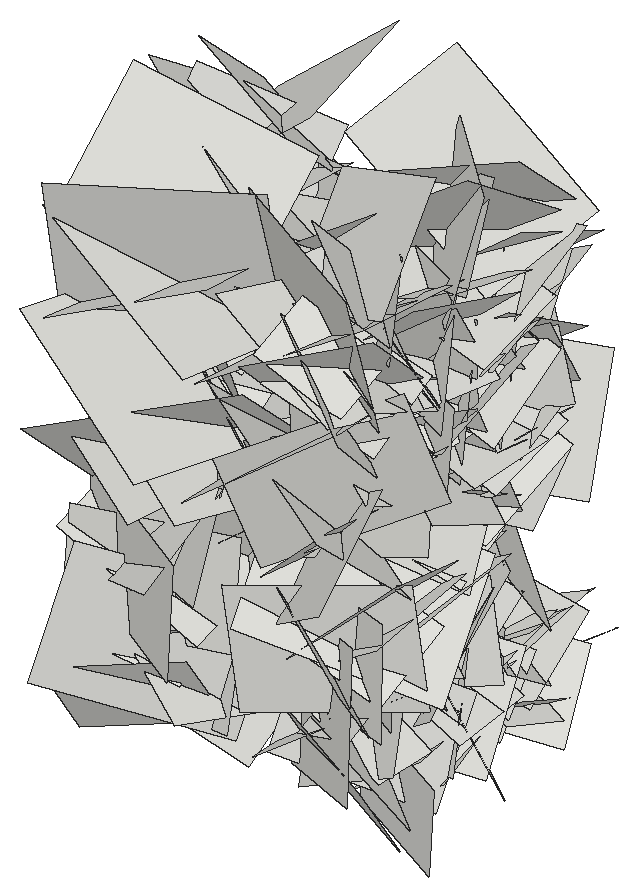
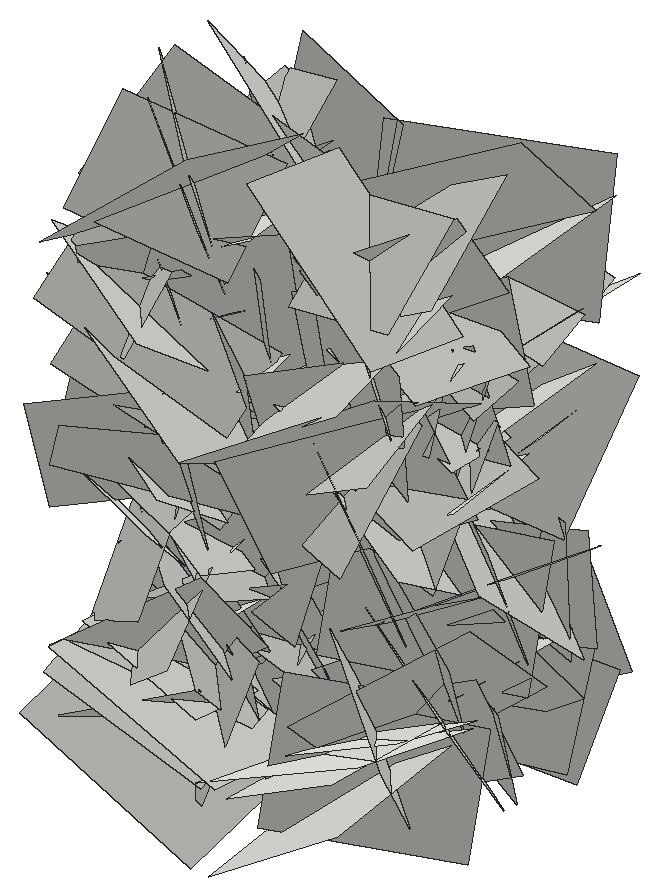
# SketchUp Ruby script. Lengths in inches.
U = 1.inch
M = Sketchup.active_model
def pt(a) = Geom::Point3d.new(a.map { |v| v * U })
def face(e, loops, mat)
  f = e.add_face(loops[0].map { |a| pt(a) })
  loops[1..].each { |l| e.add_face(l.map { |a| pt(a) }).erase! }
  f.material = f.back_material = mat if mat
  f
end
# faces: each face lists its corners as indices into pts; further lists are holes
def faces(e, pts, list, mat = nil) = list.each { |f| face(e, (f[0].is_a?(Array) ? f : [f]).map { |l| l.map { |i| pts[i] } }, mat) }
# xy, xz, yz: faces in a plane at the given z, y or x. An outline is a flat list of corners, or four numbers for a rectangle; further outlines are holes
def ring(l) = l.size == 4 ? [[l[0], l[1]], [l[2], l[1]], [l[2], l[3]], [l[0], l[3]]] : l.each_slice(2).to_a
def flat(e, list, mat, &to3) = list.each { |f| face(e, (f[0].is_a?(Array) ? f : [f]).map { |l| ring(l).map { |u, v| to3.(u, v) } }, mat) }
def xy(e, z, list, mat = nil) = flat(e, list, mat) { |x, y| [x, y, z] }
def xz(e, y, list, mat = nil) = flat(e, list, mat) { |x, z| [x, y, z] }
def yz(e, x, list, mat = nil) = flat(e, list, mat) { |y, z| [x, y, z] }
def lines(e, pts, list) = list.each { |a, b| e.add_line(pt(pts[a]), pt(pts[b])) }
# prism: a flat outline (further loops are holes) pulled along v
def prism(e, loops, v, mat = nil)
  f = face(e, loops, mat); d = Geom::Vector3d.new(v.map { |x| x * U })
  f.pushpull(f.normal.samedirection?(d) ? d.length : -d.length)
end
def box(e, o, s, mat = nil) = prism(e, [[o, [o[0] + s[0], o[1], o[2]], [o[0] + s[0], o[1] + s[1], o[2]], [o[0], o[1] + s[1], o[2]]]], [0, 0, s[2]], mat)
def at(x, y, z, deg = 0) = Geom::Transformation.translation(pt([x, y, z])) * Geom::Transformation.rotation(ORIGIN, Z_AXIS, deg.degrees)
def axes(o, x, y, z) = Geom::Transformation.new([*x, 0, *y, 0, *z, 0, *pt(o).to_a, 1])
def part(name) = M.definitions.add(name)
# library, detail: a bought-in or finely detailed component or shape, given as its bounding box
def library(name, o, s) = part(name).tap { |d| box(d.entities, o, s) }
def detail(e, o, s) = box(e.add_group.entities, o, s)
def put(e, d, t, mat = nil) = e.add_instance(d, t).tap { |i| i.material = mat if mat }
def group(e, t, mat = nil) = e.add_group.tap { |g| g.transformation = t; g.material = mat if mat }.entities
root = M.entities
c1 = part("Component\#6")
p = [[0.01,0,0],[0,3.24,4.54],[4.32,3.24,4.54],[4.33,0,0]]
faces(c1.entities,p,[[0,1,2,3]])
put(root,c1,axes([14.53,197.24,20.32],[0.11105,0.4932,0.81979],[-0.10012,0.82599,-0.48487],[1.00916,0.02768,-0.13831]))
put(root,c1,axes([14.53,196.19,13.89],[-0.03711,0.95345,-0.08325],[0.1071,-0.07916,-0.94908],[1.00884,0.04348,0.09769]))
put(root,c1,axes([18.5,198.53,13.8],[0.10676,-0.41647,0.70694],[0.09382,0.7136,0.40779],[-0.86465,0.02601,0.13154]))
put(root,c1,axes([18.5,201.03,8.02],[0.03451,-0.61291,-0.20918],[-0.0475,-0.21108,0.61149],[-0.68484,-0.01625,-0.05296]))
put(root,c1,axes([18.5,199.53,17.66],[0.07108,0.22718,0.77768],[0.14032,0.76678,-0.23541],[-0.84726,0.14605,0.02626]))
put(root,c1,axes([18.5,196.1,5.28],[0.08762,-0.56519,-0.39893],[-0.0287,-0.4041,0.56691],[-0.73275,-0.05175,-0.06991]))
put(root,c1,axes([14.53,192.44,8.79],[-0.05887,1.04295,0.25043],[0.00297,0.2509,-1.04431],[1.13694,0.05335,0.0157]))
put(root,c1,axes([14.53,193.71,0.46],[0.00413,-0.52236,0.7551],[0.18121,0.74232,0.51263],[0.95624,-0.13842,-0.10041]))
put(root,c1,axes([14.53,195.28,4.79],[0.03702,0.87634,0.85063],[-0.28559,0.83554,-0.84973],[1.26267,0.16329,-0.21713]))
put(root,c1,axes([14.53,203.91,5.3125],[0.18463,-0.58129,-0.78091],[-0.13848,-0.80009,0.56643],[1.02258,-0.00339,0.2177]))
put(root,c1,axes([14.53,198.93,5.125],[0.08676,0.85287,0.14934],[0.16568,0.13299,-0.84515],[0.90272,-0.10637,0.14076]))
put(root,c1,axes([14.53,198.84,9.75],[-0.24721,-0.9594,-0.88495],[-0.06038,-0.89063,0.98057],[1.38221,-0.2105,-0.11544]))
put(root,c1,axes([14.53,202.1,18.26],[-0.1919,-1.13475,-0.09678],[0.16378,-0.12156,1.13628],[1.19604,-0.16542,-0.17113]))
put(root,c1,axes([18.5,194.11,10.49],[0.01019,-0.66626,0.06574],[0.1187,0.06642,0.65679],[-0.69967,0.00157,0.11238]))
put(root,c1,axes([14.53,200.51,5.45],[-0.07717,-0.59417,-0.91785],[0.09928,-0.91989,0.58806],[1.15472,0.03938,-0.1119]))
put(root,c1,axes([14.53,205.24,14.9],[-0.1168,-0.46047,-1.13614],[-0.0362,-1.13913,0.465],[1.29896,-0.07315,-0.0892]))
put(root,c1,axes([14.53,194.25,1.05],[0.1707,-0.55728,0.79671],[-0.04122,0.80323,0.5697],[1.02978,0.12452,-0.10926]))
put(root,c1,axes([14.53,194.35,10.5],[-0.1187,0.07765,-1.12146],[0.14385,-1.11784,-0.09095],[1.18288,0.14373,-0.10148]))
put(root,c1,axes([14.53,197.36,24.8],[-0.09794,1.0389,-0.68546],[-0.01654,-0.68826,-1.04104],[1.31923,0.0685,-0.06394]))
put(root,c1,axes([18.5,199.74,12.37],[0.13977,-0.41949,-0.41774],[-0.0557,-0.43458,0.41982],[-0.62506,-0.05508,-0.13082]))
put(root,c1,axes([18.5,199.42,15.6],[0.03605,-0.49998,-0.38134],[0.14474,-0.36691,0.49324],[-0.65063,-0.10932,0.0886]))
put(root,c1,axes([14.53,200.08,24.34],[0.03463,0.75517,-0.67877],[0.20748,-0.67107,-0.73718],[1.05612,0.10708,0.16708]))
put(root,c1,axes([14.53,199.09,16.39],[0.13116,-1.14374,0.05938],[-0.13174,0.04596,1.1443],[1.20683,0.12933,0.11846]))
put(root,c1,axes([14.53,192.66,5.0625],[0.03803,0.06475,1.02957],[0.25075,1.00223,-0.07127],[1.06436,-0.23842,-0.02]))
put(root,c1,axes([14.53,196.53,2.03],[0.14871,0.38131,0.94323],[0.09041,0.94439,-0.39446],[1.07463,-0.13222,-0.09734]))
put(root,c1,axes([14.53,200.2,14.91],[0.20407,-0.96139,-0.18597],[0.07393,-0.17559,0.97991],[1.03533,0.20204,-0.03331]))
put(root,c1,axes([14.53,198.375,11.05],[-0.00636,-0.47599,-1.14741],[-0.03555,-1.14695,0.47597],[1.31628,-0.03327,0.00731]))
put(root,c1,axes([14.53,202.25,12.93],[-0.19135,-1.27912,0.12446],[0.2118,0.09622,1.27869],[1.34571,-0.19703,-0.18355]))
put(root,c1,axes([14.53,197.86,18.23],[0.19608,0.2602,-1.0463],[-0.01915,-1.06069,-0.26697],[1.14269,-0.06243,0.17507]))
put(root,c1,axes([14.53,197.84,4.84],[0.11369,-0.36766,-0.96616],[0.19069,-0.94989,0.38144],[1.07906,0.2066,0.03439]))
put(root,c1,axes([14.53,200.375,7.61],[0.26418,-0.51362,-0.84712],[0.05211,-0.86603,0.53955],[1.04881,0.1724,0.18657]))
put(root,c1,axes([14.53,203.04,12.11],[0.14841,-0.94408,-0.5752],[0.05434,-0.57362,0.95398],[1.17058,0.14632,0.02864]))
put(root,c1,axes([14.53,199.56,18.73],[0.07364,1.07871,-0.62029],[-0.05176,-0.61841,-1.08091],[1.31797,-0.08456,-0.00779]))
put(root,c1,axes([14.53,204.42,20.53],[0.1154,-1.25003,-0.28156],[-0.14973,-0.29256,1.24425],[1.34995,0.07441,0.16208]))
put(root,c1,axes([14.53,195.93,15.54],[0.04965,0.25406,1.2028],[0.02984,1.20314,-0.25523],[1.30276,-0.03724,-0.03999]))
put(root,c1,axes([14.53,198.85,12.57],[0.15345,0.48368,1.12599],[-0.09378,1.13498,-0.47617],[1.29562,0.02486,-0.16783]))
put(root,c1,axes([14.53,200.7,5.85],[0.20906,1.0682,-0.14016],[0.07965,-0.15578,-1.08152],[1.13921,-0.18514,0.10133]))
put(root,c1,axes([14.53,194.09,6.34],[0.25898,1.07168,-0.21064],[-0.01285,-0.21318,-1.09862],[1.15764,-0.24212,0.03493]))
put(root,c1,axes([14.53,192.7,21.39],[0.08893,0.79245,0.9015],[0.06254,0.89988,-0.79652],[1.27076,-0.09974,-0.02389]))
put(root,c1,axes([14.53,199.38,-0.0625],[0.15183,-0.50198,1.07326],[0.00307,1.08122,0.50532],[1.25594,0.05804,-0.13098]))
put(root,c1,axes([14.53,200.25,4.79],[0.06637,1.27776,-0.24675],[-0.01199,-0.2465,-1.2793],[1.3794,-0.06362,0.00075]))
put(root,c1,axes([14.53,192.73,15.73],[0.12897,1.2724,-0.23633],[-0.08155,-0.22984,-1.27707],[1.36939,-0.13352,-0.05379]))
put(root,c1,axes([14.53,200.21,21.54],[0.14018,1.21556,-0.55877],[-0.14242,-0.54659,-1.22085],[1.41094,-0.17594,-0.06772]))
put(root,c1,axes([14.53,190.45,18.05],[0.16537,1.24759,-0.14593],[-0.05265,-0.14081,-1.25691],[1.33042,-0.16065,-0.0316]))
put(root,c1,axes([14.53,190.86,3.39],[0.21383,0.32739,1.20741],[-0.09698,1.22359,-0.31649],[1.32251,0.03679,-0.21843]))
put(root,c1,axes([14.53,195.52,16.87],[0.17814,-1.09516,0.21581],[0.19304,0.24222,1.08736],[1.16734,0.12707,-0.21275]))
put(root,c1,axes([14.53,201.79,17.38],[0.19939,0.73728,-1.06028],[-0.09629,-1.06126,-0.75408],[1.36551,-0.18249,0.10164]))
put(root,c1,axes([14.53,196.26,4.8],[0.10051,-0.43998,1.12809],[0.21352,1.12151,0.42048],[1.26562,-0.15427,-0.16053]))
put(root,c1,axes([14.53,191.67,21.5],[0.0579,1.33618,-0.15223],[0.05318,-0.15428,-1.33612],[1.42453,-0.04855,0.05606]))
put(root,c1,axes([14.53,198.6875,16.83],[0.02201,1.26014,0.56955],[0.0456,0.56875,-1.25994],[1.46513,-0.03663,0.03065]))
put(root,c1,axes([14.53,196.95,13.22],[0.12152,0.35472,1.26895],[0.01769,1.27325,-0.35743],[1.39654,-0.047,-0.10589]))
put(root,c1,axes([14.53,197.84,15.77],[0.08558,0.66637,-1.22765],[0.01617,-1.23004,-0.66667],[1.48057,-0.02508,0.07824]))
put(root,c1,axes([14.53,193.34,3.5],[0.3285,0.68164,0.95344],[0.04901,0.97833,-0.71446],[1.2414,-0.219,-0.22409]))
put(root,c1,axes([14.53,192.59,17.15],[0.08597,-0.32374,1.28455],[0.18245,1.27862,0.31138],[1.3923,-0.14756,-0.12012]))
put(root,c1,axes([14.53,199.09,4.9],[0.11121,1.25407,0.182],[0.25083,0.16003,-1.23904],[1.31962,-0.1361,0.22018]))
put(root,c1,axes([14.53,194.4,9.86],[0.11876,-1.04596,0.91618],[0.1474,0.92297,1.03671],[1.46651,-0.00807,-0.1784]))
put(root,c1,axes([14.53,202.95,19.72],[0.19445,-0.3512,-1.29554],[0.25274,-1.27827,0.38028],[1.40021,0.2795,0.11127]))
put(root,c1,axes([28.31,202.95,19.72],[-0.19445,-0.3512,-1.29554],[-0.25274,-1.27827,0.38028],[-1.40021,0.2795,0.11127]))
put(root,c1,axes([28.31,194.4,9.86],[-0.11876,-1.04596,0.91618],[-0.1474,0.92297,1.03671],[-1.46651,-0.00807,-0.1784]))
put(root,c1,axes([28.31,199.09,4.9],[-0.11121,1.25407,0.182],[-0.25083,0.16003,-1.23904],[-1.31962,-0.1361,0.22018]))
put(root,c1,axes([28.31,192.59,17.15],[-0.08597,-0.32374,1.28455],[-0.18245,1.27862,0.31138],[-1.3923,-0.14756,-0.12012]))
put(root,c1,axes([28.31,193.34,3.5],[-0.3285,0.68164,0.95344],[-0.04901,0.97833,-0.71446],[-1.2414,-0.219,-0.22409]))
put(root,c1,axes([28.31,197.84,15.77],[-0.08558,0.66637,-1.22765],[-0.01617,-1.23004,-0.66667],[-1.48057,-0.02508,0.07824]))
put(root,c1,axes([28.31,196.95,13.22],[-0.12152,0.35472,1.26895],[-0.01769,1.27325,-0.35743],[-1.39654,-0.047,-0.10589]))
put(root,c1,axes([28.31,198.6875,16.83],[-0.02201,1.26014,0.56955],[-0.0456,0.56875,-1.25994],[-1.46513,-0.03663,0.03065]))
put(root,c1,axes([28.31,191.67,21.5],[-0.0579,1.33618,-0.15223],[-0.05318,-0.15428,-1.33612],[-1.42453,-0.04855,0.05606]))
put(root,c1,axes([28.31,196.26,4.8],[-0.10051,-0.43998,1.12809],[-0.21352,1.12151,0.42048],[-1.26562,-0.15427,-0.16053]))
put(root,c1,axes([28.31,201.79,17.38],[-0.19939,0.73728,-1.06028],[0.09629,-1.06126,-0.75408],[-1.36551,-0.18249,0.10164]))
put(root,c1,axes([28.31,195.52,16.87],[-0.17814,-1.09516,0.21581],[-0.19304,0.24222,1.08736],[-1.16734,0.12707,-0.21275]))
put(root,c1,axes([28.31,190.86,3.39],[-0.21383,0.32739,1.20741],[0.09698,1.22359,-0.31649],[-1.32251,0.03679,-0.21843]))
put(root,c1,axes([28.31,190.45,18.05],[-0.16537,1.24759,-0.14593],[0.05265,-0.14081,-1.25691],[-1.33042,-0.16065,-0.0316]))
put(root,c1,axes([28.31,200.21,21.54],[-0.14018,1.21556,-0.55877],[0.14242,-0.54659,-1.22085],[-1.41094,-0.17594,-0.06772]))
put(root,c1,axes([28.31,192.73,15.73],[-0.12897,1.2724,-0.23633],[0.08155,-0.22984,-1.27707],[-1.36939,-0.13352,-0.05379]))
put(root,c1,axes([28.31,200.25,4.79],[-0.06637,1.27776,-0.24675],[0.01199,-0.2465,-1.2793],[-1.3794,-0.06362,0.00075]))
put(root,c1,axes([28.31,199.38,-0.0625],[-0.15183,-0.50198,1.07326],[-0.00307,1.08122,0.50532],[-1.25594,0.05804,-0.13098]))
put(root,c1,axes([28.31,192.7,21.39],[-0.08893,0.79245,0.9015],[-0.06254,0.89988,-0.79652],[-1.27076,-0.09974,-0.02389]))
put(root,c1,axes([28.31,194.09,6.34],[-0.25898,1.07168,-0.21064],[0.01285,-0.21318,-1.09862],[-1.15764,-0.24212,0.03493]))
put(root,c1,axes([28.31,200.7,5.85],[-0.20906,1.0682,-0.14016],[-0.07965,-0.15578,-1.08152],[-1.13921,-0.18514,0.10133]))
put(root,c1,axes([28.31,198.85,12.57],[-0.15345,0.48368,1.12599],[0.09378,1.13498,-0.47617],[-1.29562,0.02486,-0.16783]))
put(root,c1,axes([28.31,195.93,15.54],[-0.04965,0.25406,1.2028],[-0.02984,1.20314,-0.25523],[-1.30276,-0.03724,-0.03999]))
put(root,c1,axes([28.31,204.42,20.53],[-0.1154,-1.25003,-0.28156],[0.14973,-0.29256,1.24425],[-1.34995,0.07441,0.16208]))
put(root,c1,axes([28.31,199.56,18.73],[-0.07364,1.07871,-0.62029],[0.05176,-0.61841,-1.08091],[-1.31797,-0.08456,-0.00779]))
put(root,c1,axes([28.31,203.04,12.11],[-0.14841,-0.94408,-0.5752],[-0.05434,-0.57362,0.95398],[-1.17058,0.14632,0.02864]))
put(root,c1,axes([28.31,200.375,7.61],[-0.26418,-0.51362,-0.84712],[-0.05211,-0.86603,0.53955],[-1.04881,0.1724,0.18657]))
put(root,c1,axes([28.31,197.84,4.84],[-0.11369,-0.36766,-0.96616],[-0.19069,-0.94989,0.38144],[-1.07906,0.2066,0.03439]))
put(root,c1,axes([28.31,197.86,18.23],[-0.19608,0.2602,-1.0463],[0.01915,-1.06069,-0.26697],[-1.14269,-0.06243,0.17507]))
put(root,c1,axes([28.31,202.25,12.93],[0.19135,-1.27912,0.12446],[-0.2118,0.09622,1.27869],[-1.34571,-0.19703,-0.18355]))
put(root,c1,axes([28.31,198.375,11.05],[0.00636,-0.47599,-1.14741],[0.03555,-1.14695,0.47597],[-1.31628,-0.03327,0.00731]))
put(root,c1,axes([28.31,200.2,14.91],[-0.20407,-0.96139,-0.18597],[-0.07393,-0.17559,0.97991],[-1.03533,0.20204,-0.03331]))
put(root,c1,axes([28.31,196.53,2.03],[-0.14871,0.38131,0.94323],[-0.09041,0.94439,-0.39446],[-1.07463,-0.13222,-0.09734]))
put(root,c1,axes([28.31,192.66,5.0625],[-0.03803,0.06475,1.02957],[-0.25075,1.00223,-0.07127],[-1.06436,-0.23842,-0.02]))
put(root,c1,axes([28.31,199.09,16.39],[-0.13116,-1.14374,0.05938],[0.13174,0.04596,1.1443],[-1.20683,0.12933,0.11846]))
put(root,c1,axes([28.31,200.08,24.34],[-0.03463,0.75517,-0.67877],[-0.20748,-0.67107,-0.73718],[-1.05612,0.10708,0.16708]))
put(root,c1,axes([24.34,199.42,15.6],[-0.03605,-0.49998,-0.38134],[-0.14474,-0.36691,0.49324],[0.65063,-0.10932,0.0886]))
put(root,c1,axes([24.34,199.74,12.37],[-0.13977,-0.41949,-0.41774],[0.0557,-0.43458,0.41982],[0.62506,-0.05508,-0.13082]))
put(root,c1,axes([28.31,197.36,24.8],[0.09794,1.0389,-0.68546],[0.01654,-0.68826,-1.04104],[-1.31923,0.0685,-0.06394]))
put(root,c1,axes([28.31,194.35,10.5],[0.1187,0.07765,-1.12146],[-0.14385,-1.11784,-0.09095],[-1.18288,0.14373,-0.10148]))
put(root,c1,axes([28.31,194.25,1.05],[-0.1707,-0.55728,0.79671],[0.04122,0.80323,0.5697],[-1.02978,0.12452,-0.10926]))
put(root,c1,axes([28.31,205.24,14.9],[0.1168,-0.46047,-1.13614],[0.0362,-1.13913,0.465],[-1.29896,-0.07315,-0.0892]))
put(root,c1,axes([28.31,200.51,5.45],[0.07717,-0.59417,-0.91785],[-0.09928,-0.91989,0.58806],[-1.15472,0.03938,-0.1119]))
put(root,c1,axes([24.34,194.11,10.49],[-0.01019,-0.66626,0.06574],[-0.1187,0.06642,0.65679],[0.69967,0.00157,0.11238]))
put(root,c1,axes([28.31,202.1,18.26],[0.1919,-1.13475,-0.09678],[-0.16378,-0.12156,1.13628],[-1.19604,-0.16542,-0.17113]))
put(root,c1,axes([28.31,198.84,9.75],[0.24721,-0.9594,-0.88495],[0.06038,-0.89063,0.98057],[-1.38221,-0.2105,-0.11544]))
put(root,c1,axes([28.31,198.93,5.125],[-0.08676,0.85287,0.14934],[-0.16568,0.13299,-0.84515],[-0.90272,-0.10637,0.14076]))
put(root,c1,axes([28.31,203.91,5.3125],[-0.18463,-0.58129,-0.78091],[0.13848,-0.80009,0.56643],[-1.02258,-0.00339,0.2177]))
put(root,c1,axes([28.31,195.28,4.79],[-0.03702,0.87634,0.85063],[0.28559,0.83554,-0.84973],[-1.26267,0.16329,-0.21713]))
put(root,c1,axes([28.31,193.71,0.46],[-0.00413,-0.52236,0.7551],[-0.18121,0.74232,0.51263],[-0.95624,-0.13842,-0.10041]))
put(root,c1,axes([28.31,192.44,8.79],[0.05887,1.04295,0.25043],[-0.00297,0.2509,-1.04431],[-1.13694,0.05335,0.0157]))
put(root,c1,axes([24.34,196.1,5.28],[-0.08762,-0.56519,-0.39893],[0.0287,-0.4041,0.56691],[0.73275,-0.05175,-0.06991]))
put(root,c1,axes([24.34,199.53,17.66],[-0.07108,0.22718,0.77768],[-0.14032,0.76678,-0.23541],[0.84726,0.14605,0.02626]))
put(root,c1,axes([24.34,201.03,8.02],[-0.03451,-0.61291,-0.20918],[0.0475,-0.21108,0.61149],[0.68484,-0.01625,-0.05296]))
put(root,c1,axes([24.34,198.53,13.8],[-0.10676,-0.41647,0.70694],[-0.09382,0.7136,0.40779],[0.86465,0.02601,0.13154]))
put(root,c1,axes([28.31,196.19,13.89],[0.03711,0.95345,-0.08325],[-0.1071,-0.07916,-0.94908],[-1.00884,0.04348,0.09769]))
put(root,c1,axes([28.31,197.24,20.32],[-0.11105,0.4932,0.81979],[0.10012,0.82599,-0.48487],[-1.00916,0.02768,-0.13831]))
put(root,c1,axes([24.34,202.56,19.21],[0.06396,-0.26998,-0.58675],[-0.04641,-0.58965,0.26682],[0.68306,-0.01478,0.07307]))
put(root,c1,axes([24.34,199.64,2.06],[-0.21894,0.61345,0.59822],[0.01858,0.61825,-0.62794],[0.90807,0.13525,0.15708]))
put(root,c1,axes([28.31,196.07,8.125],[-0.08332,-0.69698,-0.457],[-0.10667,-0.44773,0.70016],[-0.87699,0.12068,-0.04174]))
put(root,c1,axes([24.34,190.79,19.57],[0.04866,0.55121,0.30162],[0.00575,0.30207,-0.55285],[0.66601,-0.04288,-0.01726]))
put(root,c1,axes([24.34,195.85,11.01],[-0.15114,0.73817,0.19544],[0.07767,0.21113,-0.74396],[0.80568,0.11812,0.10838]))
put(root,c1,axes([28.31,202.76,13.17],[0.11284,-1.03894,-0.17524],[-0.03066,-0.17895,1.04335],[-1.11641,-0.1001,-0.04636]))
put(root,c1,axes([28.31,189.31,11.46],[-0.01967,0.80876,0.77653],[0.21901,0.76581,-0.79265],[-1.16812,0.12996,-0.16169]))
put(root,c1,axes([24.34,193.57,4.75],[0.0218,0.6351,0.02763],[0.03876,0.02642,-0.63443],[0.67273,-0.0221,0.03566]))
put(root,c1,axes([28.31,199.68,18.17],[0.10811,0.81171,0.57509],[-0.11351,0.5837,-0.80488],[-1.04835,0.0205,0.14645]))
put(root,c1,axes([24.34,202.9,8.46],[-0.28421,-0.45126,-0.90988],[-0.10984,-0.92399,0.48879],[1.07096,-0.21452,-0.19133]))
put(root,c1,axes([24.34,193.91,15.9375],[0.03263,0.61645,-0.26034],[-0.02336,-0.25954,-0.61716],[0.70894,-0.03692,-0.00835]))
put(root,c1,axes([24.34,192.26,20.51],[-0.14395,0.6641,-0.62024],[-0.10915,-0.63433,-0.65665],[0.95701,0.02754,-0.16819]))
put(root,c1,axes([24.34,199.23,1.1],[-0.00098,-0.71414,-0.15761],[-0.04174,-0.15733,0.71311],[0.77408,-0.00939,0.03826]))
put(root,c1,axes([24.34,196.5625,6.92],[0.07674,-0.09799,-0.6482],[-0.03176,-0.65195,0.09521],[0.69417,-0.019,0.07601]))
put(root,c1,axes([24.34,198.91,12.75],[-0.15355,-0.10183,1.00426],[-0.21738,0.99636,0.07145],[1.04766,0.19182,0.16201]))
put(root,c1,axes([24.34,195.68,15.75],[0.06715,-0.51242,0.33521],[0.05381,0.34023,0.51051],[0.64683,0.02489,-0.07727]))
put(root,c1,axes([24.34,200.4375,8.06],[-0.17377,0.75884,-0.49804],[-0.05898,-0.51355,-0.76415],[0.96033,0.10576,-0.13705]))
put(root,c1,axes([24.34,199.6875,17.84],[0.07891,0.44569,0.39814],[0.07493,0.39183,-0.45185],[0.62903,-0.10259,0.00388]))
put(root,c1,axes([24.34,200.03,9.27],[-0.00412,-0.60297,0.30435],[0.07057,0.30253,0.60022],[0.71247,-0.03345,-0.05769]))
put(root,c1,axes([24.34,192.95,10.8],[0.02962,0.02518,0.78508],[-0.12702,0.77652,-0.02064],[0.82287,0.11896,-0.03145]))
put(root,c1,axes([28.31,199.37,10.67],[0.09558,-1.01864,0.46326],[0.13943,0.47118,1.01047],[-1.17795,-0.02688,0.1572]))
put(root,c1,axes([24.34,198.38,4.95],[-0.02223,0.32868,-0.55446],[0.17267,-0.53404,-0.32274],[0.66105,0.15055,0.06565]))
put(root,c1,axes([24.34,192.04,10.01],[-0.12172,0.5206,-0.6372],[0.01939,-0.6416,-0.52749],[0.87198,0.08694,-0.07722]))
put(root,c1,axes([24.34,202.51,19.98],[0.06792,0.48446,-0.5602],[-0.10116,-0.55221,-0.48846],[0.77852,-0.11402,-0.01459]))
put(root,c1,axes([28.31,195.86,16.68],[-0.06531,-0.43873,0.684],[-0.07025,0.68639,0.43429],[-0.8585,-0.02279,-0.08757]))
put(root,c1,axes([24.34,202.74,-0.14],[0.03158,-0.64507,0.25861],[0.01592,0.25938,0.64528],[0.73651,0.02205,-0.02503]))
put(root,c1,axes([28.31,192.22,20.81],[-0.00161,0.62306,-0.59539],[-0.0785,-0.59329,-0.62067],[-0.91013,0.05007,0.05459]))
put(root,c1,axes([24.34,197.35,3.52],[0.03443,0.41092,0.66217],[-0.08038,0.66126,-0.40665],[0.82215,0.04744,-0.06748]))
put(root,c1,axes([24.34,195.99,4.23],[-0.18601,0.0566,0.88651],[0.05201,0.90288,-0.04793],[0.94017,-0.03875,0.17804]))
put(root,c1,axes([28.31,198.67,11.97],[0.07539,0.76068,0.50866],[-0.0723,0.51318,-0.75791],[-0.96729,0.02092,0.0963]))
put(root,c1,axes([24.34,195.9375,9.16],[0.07841,0.69576,-0.29748],[-0.09095,-0.28926,-0.69787],[0.79692,-0.10147,-0.05038]))
put(root,c1,axes([28.31,195.4375,18.11],[-0.16874,-0.51977,-0.57708],[0.05885,-0.59519,0.52076],[-0.82114,0.06415,0.15591]))
put(root,c1,axes([28.31,196.17,12.88],[0.06274,0.02618,0.84664],[-0.15393,0.83645,-0.01571],[-0.88457,-0.1437,0.06278]))
put(root,c1,axes([28.31,193.46,10.77],[-0.10152,0.90556,-0.18731],[0.17799,-0.16815,-0.89879],[-0.96391,-0.12642,-0.14624]))
put(root,c1,axes([24.34,200.82,0.59],[0.02153,-0.73416,-0.35765],[-0.0933,-0.35764,0.72915],[0.8606,-0.02041,0.08799]))
put(root,c1,axes([28.31,195.73,16.63],[0.01219,-0.78698,0.32297],[-0.05977,0.32158,0.78561],[-0.89973,-0.03203,-0.04781]))
put(root,c1,axes([28.31,196.375,20.79],[0.12547,0.87042,-0.10702],[-0.18806,-0.08199,-0.86307],[-0.91037,0.1369,0.16354]))
put(root,c1,axes([28.31,200.05,13.66],[-0.07814,0.81604,-0.08962],[0.02759,-0.08761,-0.81916],[-0.86976,-0.0761,-0.01794]))
put(root,c1,axes([28.31,198.3125,4.47],[0.08144,0.93817,-0.09306],[0.01009,-0.09413,-0.94116],[-0.99929,0.07551,-0.01709]))
put(root,c1,axes([28.31,200.41,3.58],[0.05776,-0.87144,-0.04483],[-0.06577,-0.04867,0.87073],[-0.92261,-0.05109,-0.06488]))
put(root,c1,axes([28.31,195.95,14.86],[0.17446,0.9838,0.62037],[0.19333,0.59697,-0.99508],[-1.2176,0.23574,-0.06911]))
put(root,c1,axes([28.31,194.43,21.03],[0.18864,1.08922,-0.2367],[0.12278,-0.25647,-1.09312],[-1.17512,0.14806,-0.15221]))
put(root,c1,axes([24.34,200.69,6.875],[-0.16125,-0.91938,-0.30199],[-0.04119,-0.29965,0.93182],[1.02494,-0.15668,-0.01006]))
put(root,c1,axes([28.31,193.09,19.46],[-0.07295,0.25641,0.83596],[0.12348,0.83376,-0.24615],[-0.9186,0.09171,-0.09948]))
put(root,c1,axes([28.31,196.25,20.97],[-0.03433,0.46285,-0.75346],[0.09275,-0.74858,-0.46362],[-0.93272,-0.09148,-0.01837]))
put(root,c1,axes([24.34,193.9,23.36],[0.05376,0.55183,-0.55937],[-0.04326,-0.55793,-0.55411],[0.83178,-0.06469,0.00734]))
put(root,c1,axes([28.31,193.92,18.08],[0.13809,0.41624,-1.10581],[0.27382,-1.09563,-0.38198],[-1.22215,-0.19844,-0.21052]))
put(root,c1,axes([28.31,202.38,16.09],[0.07402,-0.92988,-0.45649],[0.17154,-0.44211,0.92536],[-1.08456,-0.13339,0.1152]))
put(root,c1,axes([24.34,201.99,11.3125],[-0.07595,0.62186,-0.76254],[-0.14567,-0.76339,-0.60964],[1.03278,-0.06194,-0.14206]))
put(root,c1,axes([24.34,202.11,15.27],[0.00741,-0.76642,-0.19435],[0.02033,-0.19414,0.76626],[0.83787,0.01149,-0.01688]))
put(root,c1,axes([28.31,195.27,-1.16],[0.10176,-0.07093,0.82892],[-0.16666,0.81783,0.08819],[-0.86597,-0.16573,0.08043]))
put(root,c1,axes([28.31,196.11,19.5625],[0.1708,0.27531,1.11719],[0.21419,1.10379,-0.30115],[-1.2007,0.23607,0.1052]))
put(root,c1,axes([24.34,200.46,4.14],[0.03987,0.66432,-0.22968],[0.12809,-0.2327,-0.65325],[0.73398,0.00452,0.12648]))
put(root,c1,axes([28.31,200.85,9.74],[-0.02518,0.49854,0.49521],[-0.19267,0.47427,-0.48618],[-0.7195,-0.14445,0.11286]))
